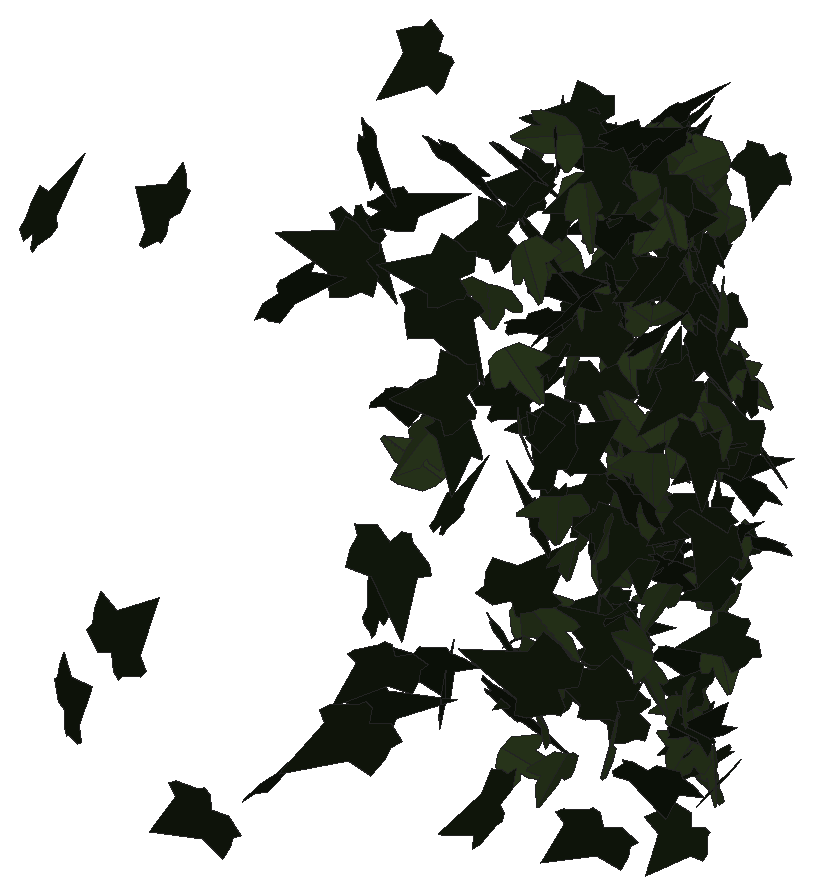
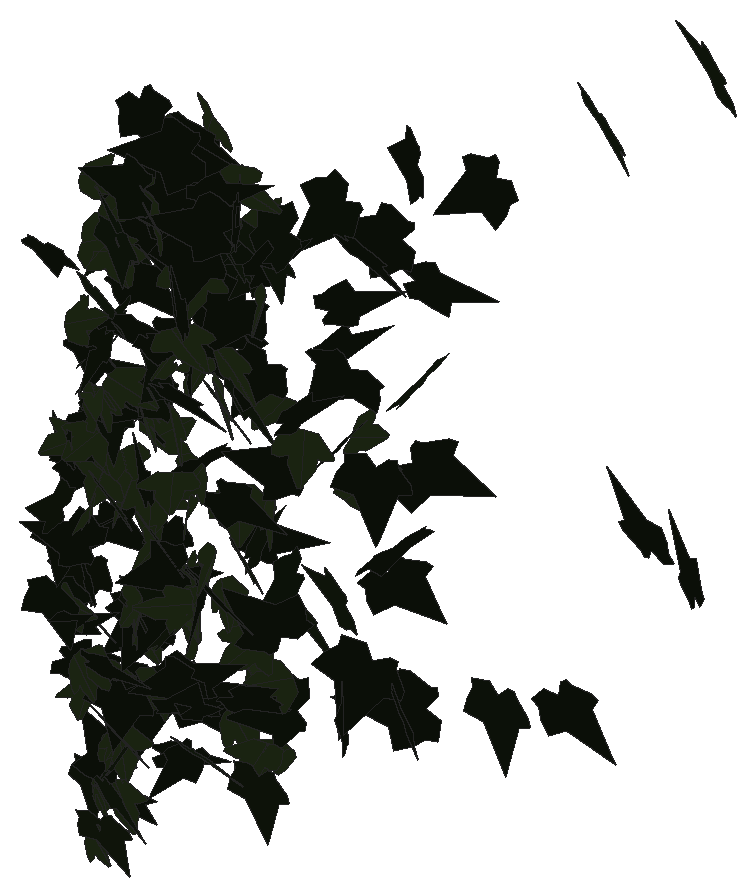
# SketchUp Ruby script. Lengths in millimetres.
U = 1.mm
M = Sketchup.active_model
def pt(a) = Geom::Point3d.new(a.map { |v| v * U })
def face(e, loops, mat)
  f = e.add_face(loops[0].map { |a| pt(a) })
  loops[1..].each { |l| e.add_face(l.map { |a| pt(a) }).erase! }
  f.material = f.back_material = mat if mat
  f
end
# faces: each face lists its corners as indices into pts; further lists are holes
def faces(e, pts, list, mat = nil) = list.each { |f| face(e, (f[0].is_a?(Array) ? f : [f]).map { |l| l.map { |i| pts[i] } }, mat) }
# xy, xz, yz: faces in a plane at the given z, y or x. An outline is a flat list of corners, or four numbers for a rectangle; further outlines are holes
def ring(l) = l.size == 4 ? [[l[0], l[1]], [l[2], l[1]], [l[2], l[3]], [l[0], l[3]]] : l.each_slice(2).to_a
def flat(e, list, mat, &to3) = list.each { |f| face(e, (f[0].is_a?(Array) ? f : [f]).map { |l| ring(l).map { |u, v| to3.(u, v) } }, mat) }
def xy(e, z, list, mat = nil) = flat(e, list, mat) { |x, y| [x, y, z] }
def xz(e, y, list, mat = nil) = flat(e, list, mat) { |x, z| [x, y, z] }
def yz(e, x, list, mat = nil) = flat(e, list, mat) { |y, z| [x, y, z] }
def lines(e, pts, list) = list.each { |a, b| e.add_line(pt(pts[a]), pt(pts[b])) }
# prism: a flat outline (further loops are holes) pulled along v
def prism(e, loops, v, mat = nil)
  f = face(e, loops, mat); d = Geom::Vector3d.new(v.map { |x| x * U })
  f.pushpull(f.normal.samedirection?(d) ? d.length : -d.length)
end
def box(e, o, s, mat = nil) = prism(e, [[o, [o[0] + s[0], o[1], o[2]], [o[0] + s[0], o[1] + s[1], o[2]], [o[0], o[1] + s[1], o[2]]]], [0, 0, s[2]], mat)
def at(x, y, z, deg = 0) = Geom::Transformation.translation(pt([x, y, z])) * Geom::Transformation.rotation(ORIGIN, Z_AXIS, deg.degrees)
def axes(o, x, y, z) = Geom::Transformation.new([*x, 0, *y, 0, *z, 0, *pt(o).to_a, 1])
def part(name) = M.definitions.add(name)
# library, detail: a bought-in or finely detailed component or shape, given as its bounding box
def library(name, o, s) = part(name).tap { |d| box(d.entities, o, s) }
def detail(e, o, s) = box(e.add_group.entities, o, s)
def put(e, d, t, mat = nil) = e.add_instance(d, t).tap { |i| i.material = mat if mat }
def group(e, t, mat = nil) = e.add_group.tap { |g| g.transformation = t; g.material = mat if mat }.entities
root = M.entities
M.materials.add("efeu1").color = [18, 25, 13]
M.materials.add("efeu2").color = [43, 57, 29]
c1 = part("ivyleaf_9")
p = [[39.1,54.8,31.7],[34.5,51.8,30.2],[-5.3,25.2,17.3],[-17.9,28.3,20.9],[-21.6,21.7,17],[-20.2,4.3,5.3],
  [-22.9,-0.3,2.5],[-17.1,-4,-0.6],[-2,-2.1,-1.2],[-0.7,-15.4,-10.1],[16.6,-22.3,-16.7],[21.1,-15.1,-12.5],
  [32.7,-10.7,-11],[46.1,-1.8,-6.6],[30.8,11.2,3.8]]
faces(c1.entities,p,[[0,1,2,3,4,5,6,7,8,9,10,11,12,13,14]],"efeu1")
c2 = part("ivyleaf_10")
p = [[0,12.8,-0.8],[-1.5,51.3,-10.9],[-4.9,51,-11.6],[-13.6,26.5,-7.3],[-13.2,15.9,-4.6],[-21.1,19.3,-7.2],
  [-29.5,16.3,-8.3],[-29.2,8.3,-6.2],[-19.7,-9.8,0.5],[-7.6,-13,4],[1,-12.2,5.8],[-0.4,51.1,-11.1],
  [-1.5,51.1,-10.9],[1,-12.4,5.9],[16.9,-12.4,3.5],[35.1,9.1,-5.1],[35,12.9,-6.1],[20.5,16.4,-4.9],
  [15.8,15,-3.8],[15.3,27.6,-7.1],[12.8,31.3,-7.8]]
faces(c2.entities,p,[[0,1,2,3,4,5,6,7,8,9,10],[11,12,0,13,14,15,16,17,18,19,20]],"efeu2")
put(root,c1,axes([129.5,174.2,1877.2],[-0.13207,0.38279,1.36931],[0.49323,-1.3083,0.39769],[1.663,0.41843,-0.00921]))
put(root,c1,axes([154.7,84.5,2581.8],[-0.63255,1.33135,0.48846],[0.17757,-0.46738,1.42838],[1.72098,0.53756,0.03215]))
put(root,c1,axes([166.5,218,1950.7],[-0.65597,0.6811,1.20334],[0.88361,-0.9611,0.86761],[1.437,0.9019,0.01581]))
put(root,c1,axes([241.3,228,2566.7],[-0.6024,1.01434,0.96562],[-0.49773,0.87529,-1.12807],[-1.63447,-0.64039,-0.01237]))
put(root,c1,axes([203.9,633.2,2368.4],[0.79015,-1.1767,-0.22257],[-0.04873,0.23166,-1.34103],[1.46022,0.64446,0.07568]))
put(root,c1,axes([241.7,630.9,1843.3],[0.0072,0.25888,1.28019],[-0.37084,1.24533,-0.25043],[-1.5497,-0.29681,0.06587]))
put(root,c1,axes([252.2,293.3,1727.7],[0.22434,0.19676,-1.31509],[-1.35654,-0.70534,-0.26101],[-0.8897,1.12506,0.06636]))
put(root,c1,axes([259.7,716.1,2582.4],[-1.51138,0.12455,-0.04238],[0.05127,-0.00572,-1.24508],[-0.1521,-1.23955,0.00149]))
put(root,c1,axes([287.2,379.8,1752.7],[-0.10669,1.35705,0.11136],[-0.02549,0.11024,-1.35979],[-1.66096,-0.08886,0.01371]))
put(root,c1,axes([319.3,502.1,2413.6],[-0.84002,-0.3639,-1.06199],[-1.02252,-0.66219,0.77031],[-0.91115,1.07862,0.11462]))
put(root,c1,axes([306.4,608.7,2184.8],[0.49177,1.18402,-0.32712],[-0.12156,-0.31163,-1.25074],[-1.49368,0.41518,-0.00591]))
put(root,c1,axes([318,776.4,2327.1],[-0.51042,-0.40932,1.02251],[-0.75578,-0.81692,-0.5805],[1.11101,-0.74378,0.07487]))
put(root,c2,axes([329.7,732.7,2273.6],[-1.39313,-0.24607,0.11644],[-0.14868,0.01308,-1.16749],[0.29699,-1.14775,-0.03827]))
put(root,c1,axes([306,514.1,1791.2],[0.52288,0.84815,-1.03236],[0.4579,0.96409,0.94788],[1.56439,-0.56568,0.06761]))
put(root,c1,axes([328.4,649.2,1996.4],[-0.56761,1.15258,0.11734],[0.03398,-0.11528,1.24282],[1.41301,0.46577,0.01725]))
put(root,c1,axes([349.9,795.3,1794.4],[-0.02386,1.17847,0.10768],[-0.15283,0.10502,-1.1722],[-1.43562,-0.03077,0.123]))
put(root,c2,axes([366.4,573.2,2111.6],[0.56577,0.75342,0.87862],[-0.62104,-0.71729,0.88377],[1.26814,-0.68741,0.04081]))
put(root,c1,axes([352.9,306.2,2466.3],[-0.2299,0.58509,-1.22323],[-0.40371,1.1778,0.61434],[1.60425,0.38024,-0.02069]))
put(root,c1,axes([328.5,497.8,2581.2],[0.2475,-0.22054,-1.30246],[1.60047,-0.12114,0.22485],[-0.18929,-1.31259,0.19809]))
put(root,c1,axes([336.6,523.4,2478.4],[0.47822,0.87634,-0.84197],[0.27866,0.8158,0.95543],[1.45621,-0.4439,0.09367]))
put(root,c1,axes([343.1,525.8,2020],[0.03284,-1.50745,-0.09192],[0.0262,0.09231,-1.50751],[1.84231,0.02556,0.02307]))
put(root,c1,axes([355.7,559.7,1859.6],[1.29978,0.91543,-0.2444],[-0.22881,-0.15674,-1.40465],[-1.13307,1.08177,0.00329]))
put(root,c1,axes([370.7,590.6,1778.7],[-0.00958,-0.02968,1.24119],[0.17325,1.23305,0.03039],[-1.50475,0.14216,-0.00441]))
put(root,c2,axes([355.8,782.4,1827],[0.71654,0.8968,0.53146],[0.22015,0.51333,-1.06564],[-1.25259,0.60323,0.11673]))
put(root,c1,axes([348.6,611.4,2320],[-0.55251,-0.44446,-1.25416],[1.23915,0.74035,-0.62914],[1.04865,-1.10901,0.08264]))
put(root,c1,axes([396.5,584.9,2381],[-0.44441,-0.16062,1.12111],[-1.26259,-0.43116,-0.39804],[0.56125,-1.09712,-0.00771]))
put(root,c2,axes([377.5,758.1,2472.3],[-0.68124,1.03577,-0.30731],[0.12435,-0.29389,-1.17571],[-1.31221,-0.56558,0.04813]))
put(root,c2,axes([387.8,544.7,2179.8],[0.23852,0.57216,-1.11063],[-0.36045,-1.07108,-0.6038],[-1.48097,0.35284,-0.03192]))
put(root,c1,axes([378.2,588.4,2548.1],[1.64541,-0.02993,-0.15899],[-0.19373,0.01054,-1.34901],[0.03776,1.35799,0.00697]))
put(root,c1,axes([409.7,447.3,1923.4],[0.02285,0.4628,-1.16576],[-0.24247,-1.15006,-0.45976],[-1.51087,0.19157,0.05615]))
put(root,c2,axes([417.4,685.9,2130.4],[-0.64652,0.4216,0.99529],[-0.90191,0.66731,-0.67628],[-0.96204,-0.90892,-0.03485]))
put(root,c1,axes([389.7,590.8,2176.8],[0.04438,-1.2495,0.4438],[0.00985,-0.44375,-1.25002],[1.61766,0.03698,-0.00456]))
put(root,c2,axes([402,832.9,2118.7],[-0.86081,0.86897,-0.0138],[0.02275,-0.00263,-1.11928],[-1.06004,-0.70571,-0.01282]))
put(root,c1,axes([435.9,833.2,1827.3],[-0.88476,0.63921,0.41019],[-0.61035,0.02469,-0.92298],[-0.69717,-0.83282,0.28747]))
put(root,c1,axes([395,664.1,2174.6],[0.2251,0.06574,1.31526],[1.41711,0.61763,-0.19382],[-0.75697,1.17579,0.02828]))
put(root,c1,axes([436,691.5,2468.2],[-0.2236,-0.19881,1.10316],[-0.95829,-0.77468,-0.27011],[0.97562,-0.80649,-0.01248]))
put(root,c2,axes([445.3,740.9,2357.5],[1.00905,-0.43387,-0.77565],[-0.81549,0.39464,-0.9335],[0.7146,1.06301,0.02997]))
put(root,c1,axes([411.4,662.6,2522.1],[1.55237,-0.37924,0.13675],[0.19419,0.05661,-1.32403],[0.45187,1.27851,0.09919]))
put(root,c1,axes([464.4,726.1,2144.1],[-0.17849,-0.04731,-1.12376],[-1.01014,-0.76247,0.1399],[-0.92874,0.83839,0.06381]))
put(root,c1,axes([454.4,526.6,2263.6],[-0.48259,-0.31287,1.22597],[-1.03679,-0.88592,-0.50029],[1.14361,-0.9352,0.06378]))
put(root,c1,axes([462,642.5,2479.3],[-0.21515,1.14308,0.65088],[-0.43793,0.58996,-1.13335],[-1.54388,-0.32664,0.23078]))
put(root,c1,axes([438.2,828.9,1816.1],[0.11107,-0.15727,-1.03371],[-0.40404,0.97986,-0.17825],[1.20997,0.34164,0.03537]))
put(root,c1,axes([427.9,657.8,1920.5],[-0.39436,-0.20959,1.28643],[1.51304,0.35822,0.37],[-0.48911,1.27713,0.10734]))
put(root,c1,axes([467.9,683.5,2033],[-0.82797,0.29001,-0.80103],[-0.91813,0.27587,0.73748],[0.48708,1.01298,0.02849]))
put(root,c1,axes([476.6,753.9,2019.4],[-0.89766,0.70353,0.66675],[-0.63436,0.41997,-1.01694],[-0.99798,-0.89976,0.04668]))
put(root,c2,axes([435.1,644.2,2255.1],[0.90488,0.55782,0.63925],[0.63054,0.37629,-0.92802],[-0.82085,0.90398,-0.00817]))
put(root,c1,axes([450.3,658,2309.7],[0.85182,0.84288,0.17455],[0.10601,0.15459,-1.09406],[-1.04477,0.7029,0.03131]))
put(root,c1,axes([424.3,630.2,1798],[1.40128,-0.56147,0.553],[0.60594,-0.24318,-1.27847],[0.74647,1.25137,-0.00032]))
put(root,c1,axes([469.9,660.1,2026.3],[0.20324,-1.0426,0.66961],[-0.13113,0.66093,1.05582],[-1.50601,-0.19825,-0.00156]))
put(root,c2,axes([439.7,636.6,1840.7],[-0.78712,0.19285,-0.96428],[1.11327,-0.31243,-0.67303],[-0.44715,-1.11735,0.02176]))
put(root,c1,axes([446.6,831.3,2446.1],[-0.0276,0.20015,1.06889],[0.26995,-1.04591,0.20053],[1.29896,0.22161,-0.01896]))
put(root,c1,axes([476.8,682.2,1821.8],[-1.10396,-0.49147,0.48713],[-0.51547,-0.24265,-1.02969],[0.66857,-0.99862,0.01046]))
put(root,c2,axes([448.6,630,1724.9],[0.32908,0.62154,0.87728],[0.40318,0.81275,-0.67743],[-1.24817,0.4264,0.01248]))
put(root,c1,axes([472.3,734.4,2293.1],[-1.19011,0.33031,-0.36441],[0.4097,-0.14406,-1.02955],[-0.4384,-1.03133,0.0271]))
put(root,c1,axes([455.3,713.1,2527.9],[0.03084,0.223,1.25674],[-0.17841,-1.24821,0.22442],[1.54692,-0.1484,0.00083]))
put(root,c2,axes([447.7,834.6,2035.2],[-0.04776,0.00827,-1.09935],[1.01199,0.72216,-0.0241],[0.88024,-0.82981,-0.03194]))
put(root,c1,axes([484.3,679,2278.6],[-1.20077,0.71194,-0.38246],[0.36061,-0.24381,-1.21452],[-0.91765,-1.02741,0.02319]))
put(root,c1,axes([453.9,837.5,2003.5],[0.65248,-0.95946,-0.06539],[-0.03845,0.0573,-1.09845],[1.17262,0.53575,0.00037]))
put(root,c2,axes([494.8,670.6,2572.3],[0.62219,0.05024,-1.12526],[-1.37358,0.05956,-0.50762],[0.04096,1.234,0.07032]))
put(root,c2,axes([464.6,666.6,1899.2],[-1.1716,-0.08304,-0.64359],[0.78655,0.00878,-0.96313],[0.09014,-1.15601,0.03892]))
put(root,c2,axes([479.9,705,1989],[-0.09347,-1.06379,-0.08029],[0.02137,0.07924,-1.06648],[1.30134,-0.07771,0.01174]))
put(root,c1,axes([500.3,725,2568.2],[-0.50526,-0.24688,1.06482],[-1.16638,-0.47018,-0.48085],[0.64645,-1.0413,-0.03533]))
put(root,c2,axes([474.3,817.8,2203.9],[0.91303,0.87208,0.04465],[0.03806,0.03207,-1.14917],[-1.06465,0.74903,-0.00279]))
put(root,c2,axes([486,801,2284.4],[0.92984,-0.8197,-0.34255],[-0.1361,0.35946,-1.10837],[1.07526,0.75434,0.15593]))
put(root,c1,axes([468.6,636.1,2448.5],[1.32723,-0.68166,-0.25782],[-0.25148,0.15652,-1.28361],[0.85281,1.10702,0.02273]))
put(root,c1,axes([492.4,730.4,2001.5],[0.51107,-0.2919,-1.07463],[-1.07735,0.61238,-0.51058],[0.82764,0.9774,-0.00104]))
put(root,c2,axes([497,756.1,2114.7],[-0.29742,0.88332,-0.61648],[-0.17096,0.60069,0.91612],[1.30298,0.28044,-0.02052]))
put(root,c2,axes([491.1,701,2276.4],[0.95091,-0.99061,-0.05594],[-0.03916,0.04592,-1.26048],[1.20983,0.78009,0.00317]))
put(root,c1,axes([508.9,786.4,2309.9],[-1.43719,0.01297,0.11527],[-0.14142,-0.08817,-1.17473],[-0.00523,-1.18036,0.08902]))
put(root,c1,axes([499.4,669.6,2471],[-1.10052,0.44261,-0.47873],[0.49999,-0.25067,-1.004],[-0.61863,-0.98999,0.04018]))
put(root,c1,axes([467.5,817.7,2072.6],[1.16253,-0.09324,0.45213],[0.54947,-0.03986,-0.95744],[0.12362,1.05397,0.00379]))
put(root,c2,axes([512.3,602.4,1807.3],[0.37708,0.1469,-1.17444],[-0.8,1.03176,-0.04353],[1.20211,0.64055,0.33944]))
put(root,c2,axes([501.2,770.8,2386.7],[1.17472,0.50198,-0.52091],[-0.59736,-0.18614,-1.08447],[-0.64967,1.07882,0.05526]))
put(root,c1,axes([468.1,728.9,2534.7],[0.68429,0.11298,1.11735],[1.33982,0.20601,-0.57212],[-0.28653,1.23314,-0.00679]))
put(root,c1,axes([484.2,752.5,2202],[0.00626,-1.21542,-0.23705],[0.0838,0.23697,-1.21351],[1.50843,-0.00812,0.0684]))
put(root,c1,axes([498.3,739.7,2502.8],[1.23588,0.59065,-0.46052],[-0.5358,-0.15903,-1.17003],[-0.74016,1.10136,0.07802]))
put(root,c1,axes([524.9,738,1853.4],[-0.15462,0.15204,1.14733],[-1.40913,0.0567,-0.1351],[-0.08969,-1.15292,0.14466]))
put(root,c1,axes([486.9,552.3,1942.5],[1.32534,-0.51397,-0.3688],[-0.39995,0.16939,-1.20173],[0.66005,1.13466,0.01235]))
put(root,c1,axes([515.4,754.7,1819.3],[-1.18087,-0.41752,0.2475],[0.27647,0.09952,1.05413],[-0.52364,0.9941,-0.00158]))
put(root,c2,axes([510.4,639.2,2085.9],[-0.9546,-0.96482,-0.0071],[0.00105,0.00844,-1.24222],[1.17712,-0.78245,-0.00465]))
put(root,c1,axes([496.9,646.3,2383.2],[1.25881,0.76814,0.0973],[0.0823,0.07232,-1.28622],[-0.94102,1.03386,0.01767]))
put(root,c2,axes([498.6,739.1,2171.9],[-1.05849,0.5641,-0.45871],[0.42871,-0.29988,-1.03343],[-0.77654,-0.93447,0.05474]))
put(root,c2,axes([500.2,717,2327.9],[0.15996,1.12412,0.39688],[0.07064,0.3928,-1.13169],[-1.45268,0.14289,-0.01133]))
put(root,c2,axes([511.3,734.9,2461.4],[-1.34685,-0.57475,-0.03307],[0.04144,0.00636,-1.24459],[0.70113,-1.10446,0.01004]))
put(root,c1,axes([530.7,762.2,1752.6],[-0.54985,-0.50246,-0.75358],[-0.62158,-0.55528,0.67495],[-0.91359,0.68021,-0.00567]))
put(root,c2,axes([506.3,613.6,1894],[-1.43685,0.25113,-0.20413],[0.24716,-0.0287,-1.20414],[-0.3079,-1.19496,-0.01398]))
put(root,c2,axes([526,767.4,2021.6],[-1.24579,-0.04034,0.60947],[-0.74174,-0.04683,-1.02175],[0.07153,-1.18827,0.01958]))
put(root,c1,axes([527,250.3,1958.8],[-0.21417,0.07907,-1.48318],[-0.10112,-1.4917,-0.06971],[-1.80923,0.07402,0.17947]))
put(root,c1,axes([533.8,786.6,2091.1],[-0.63196,0.71169,0.61535],[-0.43613,0.50089,-0.88023],[-1.06173,-0.62936,-0.0047]))
put(root,c2,axes([522.5,831.9,1987.3],[0.13932,-0.05359,-1.06829],[-0.36353,1.03024,-0.08353],[1.25329,0.30479,0.09453]))
put(root,c2,axes([504.5,731.4,1940.6],[-0.04024,-0.33621,-0.99543],[0.35268,-0.96038,0.3148],[-1.23235,-0.26387,0.12259]))
put(root,c2,axes([514.6,719.4,1973.7],[-0.0841,0.86156,0.82187],[-0.13483,0.81506,-0.8637],[-1.44638,-0.12608,0.03272]))
put(root,c1,axes([506.9,744.5,1865.8],[0.10171,0.46391,-0.91226],[0.06561,0.91203,0.4687],[1.24687,-0.08583,0.04975]))
put(root,c2,axes([514.8,734.3,2009.8],[-0.01166,0.36078,-0.96223],[0.0046,-0.96225,-0.36082],[-1.25371,-0.00688,0.00762]))
put(root,c1,axes([536.8,770.5,2378.1],[-0.11694,-0.0803,-1.11108],[-0.43681,-1.05379,0.10705],[-1.28694,0.36497,0.06462]))
put(root,c1,axes([546.4,699,1805.4],[-0.26493,0.03685,1.14232],[-1.39134,0.06941,-0.21904],[-0.09162,-1.1607,0.02317]))
put(root,c1,axes([533.5,718.9,2356.1],[0.53279,-0.08954,-1.05895],[-1.27826,0.15523,-0.44523],[0.21687,1.1349,-0.02265]))
put(root,c2,axes([527.4,621.7,1745.5],[-0.24802,-1.07425,0.46882],[-0.05122,-0.46884,-1.0925],[1.42904,-0.20324,0.04221]))
put(root,c1,axes([547.2,699.5,2317.4],[-1.52518,0.09088,0.3312],[-0.40669,-0.02029,-1.25271],[-0.1008,-1.29311,0.04293]))
put(root,c1,axes([501.5,806.4,2027.9],[0.8715,-0.84859,0.27157],[0.24473,-0.18596,-1.10875],[1.0591,0.74125,0.03274]))
put(root,c1,axes([523.4,747.9,2011.2],[-0.72088,-1.02463,0.00589],[-0.00329,-0.00524,-1.1828],[1.25006,-0.59089,0.00028]))
put(root,c2,axes([524.8,832.7,2010.3],[-0.83051,0.69399,-0.45796],[0.38459,-0.33227,-0.9721],[-0.93867,-0.75016,0.00691]))
put(root,c2,axes([528.8,557.9,2470.2],[0.18887,1.18767,0.14534],[0.0281,0.14356,-1.19771],[-1.45949,0.15646,-0.00425]))
put(root,c1,axes([534,769.6,2008.6],[-0.51987,-1.07799,-0.26982],[0.18694,0.22922,-1.15777],[1.34277,-0.44927,0.05672]))
put(root,c1,axes([550.8,732.3,2070.9],[0.86292,0.21544,-0.83386],[-0.98956,-0.19609,-0.73869],[-0.35321,1.07571,0.03234]))
put(root,c1,axes([542.5,778.3,1966.4],[0.69472,1.01131,0.19538],[0.12181,0.16801,-1.1606],[-1.25069,0.57811,-0.0045]))
put(root,c2,axes([547.5,751.9,2306.9],[-0.34335,0.80193,0.62741],[0.04818,-0.64185,0.8381],[1.24127,0.24674,0.14101]))
put(root,c1,axes([559.5,828.6,2540.5],[-0.1559,0.96242,0.39875],[-0.13236,0.38726,-0.96946],[-1.26404,-0.15925,0.05233]))
put(root,c2,axes([537.1,662.7,2521.6],[1.27099,0.53941,0.32806],[0.28972,0.2517,-1.16798],[-0.71367,1.06283,0.1101]))
put(root,c1,axes([573.2,858.8,1915.5],[-0.8576,0.2422,0.61954],[-0.74633,0.11866,-0.74049],[-0.31876,-0.92946,0.06691]))
put(root,c2,axes([535.5,776.3,2533.1],[-0.39278,0.00342,-1.03168],[0.59731,-0.95079,-0.15594],[-1.1079,-0.51382,0.28169]))
put(root,c1,axes([537.1,793.9,2149.4],[-0.16594,0.29039,1.02051],[0.29963,-0.99231,0.3151],[1.2593,0.27437,0.0595]))
put(root,c1,axes([557.7,736.2,2297.4],[0.14861,0.64793,0.94157],[0.14801,0.93423,-0.65857],[-1.38654,0.16917,0.03062]))
put(root,c2,axes([555,776.9,2262.5],[0.6812,-1.05143,0.14462],[0.09005,-0.12455,-1.19047],[1.29168,0.56317,0.00672]))
put(root,c2,axes([572.5,808.4,2307.3],[-0.45319,-0.48566,0.8732],[-0.67854,-0.67341,-0.61115],[1.01267,-0.66856,-0.01873]))
put(root,c1,axes([575.1,829.4,1719.6],[-0.97212,0.75112,-0.0469],[0.01985,-0.0511,-1.09472],[-0.91793,-0.79656,0.026]))
put(root,c1,axes([579.1,825.8,2152.8],[-0.40786,0.68735,0.69702],[-0.48069,0.57977,-0.76071],[-1.09328,-0.51134,0.07444]))
put(root,c1,axes([544.2,766.4,1959.3],[1.29976,0.43481,0.20912],[0.24216,0.06704,-1.15062],[-0.53651,1.08363,-0.01273]))
put(root,c2,axes([563.3,741.2,2046.5],[-0.13978,0.38946,1.08071],[-0.36727,1.03794,-0.40596],[-1.35249,-0.3221,-0.00146]))
put(root,c1,axes([579.7,834.3,1666.6],[-0.28847,1.04066,0.13985],[-0.46935,0.04753,-1.00408],[-1.19194,-0.27057,0.36153]))
put(root,c1,axes([568.1,775.8,1971.2],[-0.71933,0.71077,-0.37211],[-0.37396,0.22718,0.91964],[0.90453,0.65916,0.08428]))
put(root,c2,axes([584.6,842.4,1901.7],[0.07715,0.05747,1.00865],[-1.17067,-0.31278,0.07798],[0.38563,-0.96101,0.03493]))
put(root,c2,axes([576.4,806.7,1701.4],[-1.19057,-0.08078,0.50102],[-0.57531,-0.25696,-0.95994],[0.22881,-1.06646,0.19335]))
put(root,c1,axes([549.5,741.9,2271],[0.22448,1.09586,-0.16465],[0.03085,0.16271,1.1112],[1.3516,-0.18572,0.00198]))
put(root,c2,axes([571.5,766.5,1930],[-0.26908,-1.0161,0.43504],[-0.11794,-0.42418,-1.03976],[1.34332,-0.24078,-0.00415]))
put(root,c2,axes([572.1,743.4,2119.3],[-1.27358,-0.67789,0.02379],[0.03525,-0.08806,-1.24148],[0.82678,-1.04047,0.08958]))
put(root,c1,axes([578.5,556.5,2400.6],[0.09009,1.31074,0.52223],[0.0514,0.52066,-1.31277],[-1.72059,0.08419,-0.01188]))
put(root,c2,axes([557.9,742.8,1835.1],[-1.05489,0.48843,-0.58878],[0.59398,-0.33403,-0.9921],[-0.71989,-0.99133,0.04419]))
put(root,c1,axes([595.6,415.9,1802.2],[-1.33052,1.02972,0.10081],[-0.09754,0.06216,-1.49987],[-1.25849,-1.09347,0.00967]))
put(root,c2,axes([586.2,704.3,2179],[1.00373,0.29156,0.77588],[-0.88067,-0.28519,0.87262],[0.49693,-1.09432,-0.02069]))
put(root,c2,axes([570.8,795.9,2149.9],[-0.8228,0.96065,0.08902],[-0.04594,0.08233,-1.17364],[-1.17611,-0.67528,-0.01644]))
put(root,c2,axes([591.9,838.5,1642.7],[-0.30476,0.08231,0.88203],[-1.02916,0.25766,-0.26296],[-0.32993,-0.87977,0.00551]))
put(root,c2,axes([580,795,1771.4],[-0.64418,-0.96958,0.06158],[-0.04139,-0.05165,-1.10402],[1.18454,-0.52908,-0.00508]))
put(root,c1,axes([582.9,800.5,2393.8],[-1.25614,-0.46391,-0.08687],[0.09742,0.03424,-1.12931],[0.56751,-1.03271,0.00158]))
put(root,c1,axes([576.4,789.8,1841.9],[0.78711,0.78827,-0.27102],[-0.22202,-0.20124,-1.01855],[-0.99241,0.67022,0.01291]))
put(root,c1,axes([598.7,799.7,1794],[-0.79524,0.66921,0.43797],[-0.43789,0.26014,-0.93169],[-0.87197,-0.74097,0.06846]))
put(root,c1,axes([565,688,2523.1],[1.00176,0.7523,0.49304],[-0.43568,-0.34005,1.11361],[1.00716,-0.89537,-0.00867]))
put(root,c1,axes([615.6,498.8,1933.4],[-0.6779,0.09318,1.33177],[-1.58798,0.28283,-0.56287],[-0.36203,-1.41505,-0.02481]))
put(root,c1,axes([569.3,797.5,2508.2],[-0.19713,0.87463,0.66358],[0.15723,-0.65098,0.88941],[1.33014,0.20657,-0.00679]))
put(root,c1,axes([583.9,741.9,2216.2],[-1.09797,0.70578,0.14142],[0.11574,-0.10814,1.14341],[0.8705,0.90458,0.02635]))
put(root,c1,axes([570.2,766,2577.8],[0.12685,1.06265,-0.44322],[0.03441,0.44254,1.06764],[1.40426,-0.10684,0.01387]))
put(root,c2,axes([586,795.2,1780.9],[-0.24476,1.04503,0.32623],[-0.25799,0.28842,-1.05397],[-1.31046,-0.25197,0.14656]))
put(root,c2,axes([585.6,794.2,2486.4],[0.88948,0.76062,-0.27727],[-0.25365,-0.18471,-1.05339],[-0.95456,0.75784,0.02155]))
put(root,c1,axes([580.6,816.4,1739.2],[0.70591,-0.71476,-0.53919],[0.40904,-0.42229,0.9196],[-1.01281,-0.66872,-0.00441]))
put(root,c1,axes([570.1,667.6,2589.1],[0.22782,0.88779,-0.93503],[0.22739,0.91628,0.90721],[1.5565,-0.26381,0.00432]))
put(root,c1,axes([615.9,502.1,2236.6],[-0.33394,0.74434,1.24374],[-0.65886,1.12222,-0.79047],[-1.64102,-0.60203,0.06427]))
put(root,c1,axes([604.8,708.7,2502.5],[0.06159,1.02371,-0.61251],[-0.114,-0.60778,-1.02351],[-1.45094,0.09121,0.05442]))
put(root,c2,axes([575.4,758.6,2566.6],[1.09768,0.00361,0.67761],[0.82659,-0.02266,-0.89952],[0.01311,1.12613,-0.02028]))
put(root,c2,axes([576.9,852,2278.1],[-0.25471,-0.17529,0.98399],[1.11067,-0.44822,0.11331],[0.50325,0.90051,0.24794]))
put(root,c2,axes([599.7,853.8,1900.1],[0.03265,-1.03174,0.3227],[0.0231,-0.3223,-1.03204],[1.31865,0.0312,0.01009]))
put(root,c1,axes([617.4,860.2,1958.2],[-0.81251,-0.63814,-0.34944],[-0.30914,-0.24063,0.92237],[-0.83204,0.71257,-0.00146]))
put(root,c2,axes([598.8,765.8,2171.2],[0.69404,1.03387,-0.28],[-0.2473,-0.2074,-1.17763],[-1.28314,0.59918,0.07552]))
put(root,c2,axes([585.7,825.7,2171.3],[1.23414,-0.02279,0.45663],[0.55777,0.05924,-1.00986],[-0.00443,1.1083,0.06337]))
put(root,c2,axes([589.6,844.2,2237.9],[-1.05155,0.07026,-0.57313],[0.6923,-0.08745,-0.8641],[-0.13033,-1.03138,0.03423]))
put(root,c1,axes([590,843.6,2003.9],[-0.11363,0.39556,0.91782],[0.22944,-0.8984,0.40627],[1.19753,0.20966,0.00925]))
put(root,c1,axes([599,804.4,2366],[1.02814,-0.25468,-0.66578],[-0.76341,0.22948,-0.87984],[0.41654,1.0492,0.03083]))
put(root,c2,axes([604.8,857,2406.8],[0.03752,-0.13636,1.04254],[0.05282,-1.04194,-0.13755],[1.28165,0.04694,-0.02485]))
put(root,c1,axes([629,606.2,2581.8],[-1.56321,0.20525,0.34024],[-0.40997,0.05333,-1.29765],[-0.25872,-1.32465,0.00048]))
put(root,c2,axes([598.1,837.6,2124.9],[-0.13435,0.92953,-0.41055],[0.07163,-0.40644,-0.93598],[-1.23764,-0.12443,-0.00961]))
put(root,c1,axes([616.1,822.1,2257.8],[-0.05221,-0.39228,-1.00743],[-0.18191,-0.99644,0.39433],[-1.30634,0.15443,-0.01465]))
put(root,c2,axes([601.9,814.8,2286.5],[1.27567,-0.38425,-0.06456],[-0.07007,0.03085,-1.11396],[0.47017,1.04716,0.00913]))
put(root,c1,axes([587.9,794.8,1730],[0.97198,0.72863,0.15584],[-0.14228,-0.1034,1.07965],[0.89783,-0.80519,0.00238]))
put(root,c1,axes([616.8,773.8,2249.4],[-0.07148,1.13142,0.11503],[-0.0303,0.11388,-1.13278],[-1.38711,-0.06079,0.01882]))
put(root,c1,axes([624.5,712.5,2408.2],[0.12219,0.18581,-1.08768],[-0.75742,-0.8934,-0.20979],[-1.11291,0.62843,0.02335]))
put(root,c2,axes([626.8,842.6,1974.4],[0.37691,0.01976,0.98603],[-1.19548,0.12298,0.30456],[-0.13604,-1.02595,0.0555]))
put(root,c2,axes([602.4,744.6,2550.8],[-1.11518,-0.28545,-0.69087],[0.81735,0.17123,-0.95716],[0.40451,-1.13293,0.02941]))
put(root,c1,axes([636.6,563,1720.4],[0.23388,0.31235,-1.19576],[-0.83065,-0.98318,-0.36597],[-1.25834,0.70707,0.01934]))
put(root,c1,axes([638,803.1,1955.9],[-1.09075,0.55615,0.13958],[-0.1587,0.05508,-1.0527],[-0.6813,-0.90321,0.02175]))
put(root,c1,axes([608.6,759.8,2374.7],[1.03586,-0.57421,-0.6663],[-0.52692,0.53459,-1.01108],[0.93483,0.9376,0.16842]))
put(root,c1,axes([595.4,845.2,2076.4],[0.44489,-0.08386,0.99699],[1.21516,0.13063,-0.35333],[-0.11526,1.05352,0.12317]))
put(root,c2,axes([605.8,810.7,1696.3],[0.77505,-0.51014,0.71497],[0.76576,-0.35354,-0.80997],[0.74953,0.8887,0.08819]))
put(root,c1,axes([635.9,764.6,2068.4],[0.09347,0.15798,-1.08843],[-0.41704,-1.03361,-0.17408],[-1.27535,0.34957,-0.02284]))
put(root,c2,axes([635.5,764.4,2472.6],[-0.86096,-0.58402,0.64235],[-0.50907,-0.49775,-0.91096],[0.92879,-0.81418,0.09615]))
put(root,c1,axes([642.8,769.1,2404.2],[-0.55806,0.81924,0.50508],[-0.39818,0.39405,-0.93472],[-1.10458,-0.55594,0.08177]))
put(root,c2,axes([616.5,815.4,1850.8],[0.42114,1.0868,0.09367],[0.03207,0.08993,-1.1403],[-1.33043,0.34619,0.00216]))
put(root,c1,axes([635,733.2,2254.8],[-1.40668,0.17909,-0.33272],[0.35658,-0.2544,-1.14981],[-0.29215,-1.17278,0.19861]))
put(root,c1,axes([626.7,580.1,2539.2],[0.79591,0.9812,-0.31935],[-0.22977,-0.25825,-1.17821],[-1.23772,0.67889,0.01337]))
put(root,c1,axes([601.7,532.6,2234.3],[-0.37759,-0.0444,1.23471],[1.4481,-0.36398,0.28444],[0.41837,1.21976,0.12982]))
put(root,c1,axes([633.6,733.9,1643.9],[-1.10573,-0.44663,0.02255],[-0.02362,-0.01173,-1.01041],[0.54507,-0.90654,0.00196]))
put(root,c2,axes([610,562.8,2575.3],[1.1247,-0.37775,0.74099],[0.83495,-0.28405,-0.99627],[0.5766,1.14815,-0.00269]))
put(root,c1,axes([643.5,846.4,1996.4],[0.49988,0.81496,-0.59134],[-0.80442,-0.26533,-0.82254],[-0.92839,0.6687,0.39431]))
put(root,c1,axes([618.4,730.1,2506.1],[-0.29352,-1.01985,-0.55151],[0.2523,0.51648,-1.04528],[1.39181,-0.3087,0.07318]))
put(root,c1,axes([636.2,688.8,2556.8],[-1.05525,-0.90752,0.18303],[-0.12592,-0.15439,-1.2533],[1.12243,-0.87052,0.03147]))
put(root,c1,axes([637.3,791.3,2015.2],[0.36552,1.11838,0.22488],[0.06758,0.21797,-1.15781],[-1.39009,0.30467,0.00284]))
put(root,c2,axes([635.2,793.3,2491.9],[0.0118,0.34776,-1.11875],[-0.35707,-1.08259,-0.33905],[-1.38397,0.28228,0.07794]))
put(root,c1,axes([629.4,801.1,2335.4],[-1.00698,-0.25972,-0.64052],[0.72987,0.23118,-0.86467],[0.4223,-1.01887,-0.03292]))
put(root,c2,axes([650.1,774.2,2182.7],[0.74484,-0.35892,-0.83766],[-0.79618,0.53156,-0.70341],[0.77602,0.88987,0.08232]))
put(root,c2,axes([639.8,571,1803.8],[0.71703,-0.78481,0.74131],[-0.54729,0.59019,0.98048],[-1.19798,-0.73936,-0.00423]))
put(root,c1,axes([646,773,1689.5],[-0.13477,0.92219,0.33804],[-0.04015,0.33651,-0.92876],[-1.1976,-0.11506,-0.00691]))
put(root,c1,axes([607.4,715.6,2477.7],[0.11446,-0.04199,1.23627],[1.17129,-0.77931,-0.09933],[0.95159,0.96428,-0.02644]))
put(root,c1,axes([650.2,815,1877.6],[-0.19078,-0.3981,-0.89438],[-0.18974,-0.88412,0.42072],[-1.17919,0.20667,0.077]))
put(root,c1,axes([639.1,832.4,2078.4],[0.93952,0.41199,-0.49515],[-0.55905,-0.192,-0.87243],[-0.55229,0.89519,0.04077]))
put(root,c2,axes([625,729.2,2451.3],[-0.58211,0.40722,-0.91919],[0.60201,-0.79161,-0.60684],[-1.06863,-0.66777,0.15884]))
put(root,c1,axes([656.8,683.5,2442.9],[-1.14901,0.79963,-0.20285],[0.18869,-0.13126,-1.23548],[-0.98861,-0.95442,-0.00004]))
put(root,c1,axes([654.8,781,2154.2],[0.05656,0.2626,-1.04836],[-0.28386,-1.02229,-0.26636],[-1.2876,0.23691,0.01267]))
put(root,c2,axes([664.4,605.8,1956.1],[0.32936,-0.2654,-1.16824],[-1.08826,0.75487,-0.37762],[0.97565,0.93159,-0.02683]))
put(root,c2,axes([620.7,832.1,2218.6],[0.67675,0.2393,0.88076],[0.92659,0.45052,-0.60075],[-0.61747,0.93834,0.06382]))
put(root,c1,axes([652.8,821.4,2191.7],[0.28324,-0.12038,0.98571],[-0.31348,0.97053,0.17905],[-1.17024,-0.28912,0.19062]))
put(root,c1,axes([646.6,642.7,1764.9],[1.22102,0.68551,-0.53387],[-0.54479,-0.29276,-1.21305],[-0.90932,1.09589,0.00989]))
put(root,c2,axes([647.4,638.6,2560.3],[0.01237,-0.20831,1.1603],[0.09758,-1.15755,-0.20851],[1.43489,0.08052,0.00418]))
put(root,c1,axes([626.1,860,2126.8],[0.7527,-0.7067,0.39551],[0.30142,-0.30925,-0.93798],[0.94091,0.6644,-0.01591]))
put(root,c2,axes([652.9,658.4,2523.5],[1.38784,0.04284,-0.42704],[-0.52051,-0.01851,-1.13838],[-0.05686,1.21495,-0.00228]))
put(root,c1,axes([658.3,653.8,2626.2],[-0.32618,1.00407,-0.63107],[0.24142,-0.60007,-1.03858],[-1.42654,-0.33114,-0.03146]))
put(root,c1,axes([638.1,748.4,2309.6],[0.74691,-0.79634,-0.50815],[-0.3913,0.39433,-1.0044],[1.08402,0.69104,-0.01243]))
put(root,c2,axes([658.5,754.2,2561],[-0.3003,-0.15816,1.04049],[-0.28818,-1.03301,-0.2129],[1.25122,-0.27588,0.20069]))
put(root,c1,axes([664.9,788,2152.6],[-1.24641,-0.43663,0.11309],[0.13548,0.0279,1.1109],[-0.53333,1.02751,0.0179]))
put(root,c2,axes([660.8,660,2533.3],[-0.82502,0.82142,0.54961],[-0.58843,0.30698,-1.05225],[-1.05243,-0.81556,0.15748]))
put(root,c1,axes([639.7,750.8,2171.6],[0.04017,-1.17597,0.1897],[-0.03348,-0.19047,-1.17598],[1.45284,0.02813,-0.03235]))
put(root,c1,axes([649.7,864.5,2508.4],[-0.98307,-0.34404,-0.49094],[0.59396,0.10436,-0.87222],[0.42675,-0.93778,0.08304]))
put(root,c2,axes([662.3,764.9,2368.1],[-0.77447,0.9004,0.31517],[-0.58952,0.02292,-1.03876],[-1.00349,-0.70837,0.367]))
put(root,c1,axes([639,754.6,2448.5],[0.16419,-0.89301,0.59242],[0.18573,-0.57509,-0.90147],[1.29415,0.19583,0.05421]))
put(root,c1,axes([647.7,770,2046.2],[-0.43814,-1.04313,0.34089],[0.06117,-0.3739,-1.09132],[1.33745,-0.32462,0.16158]))
